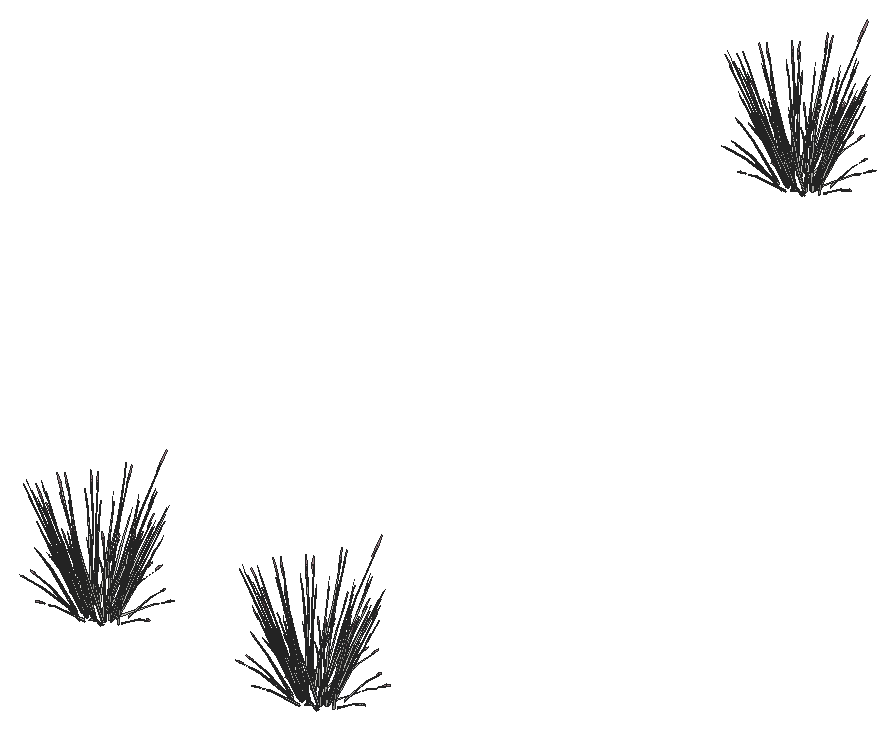
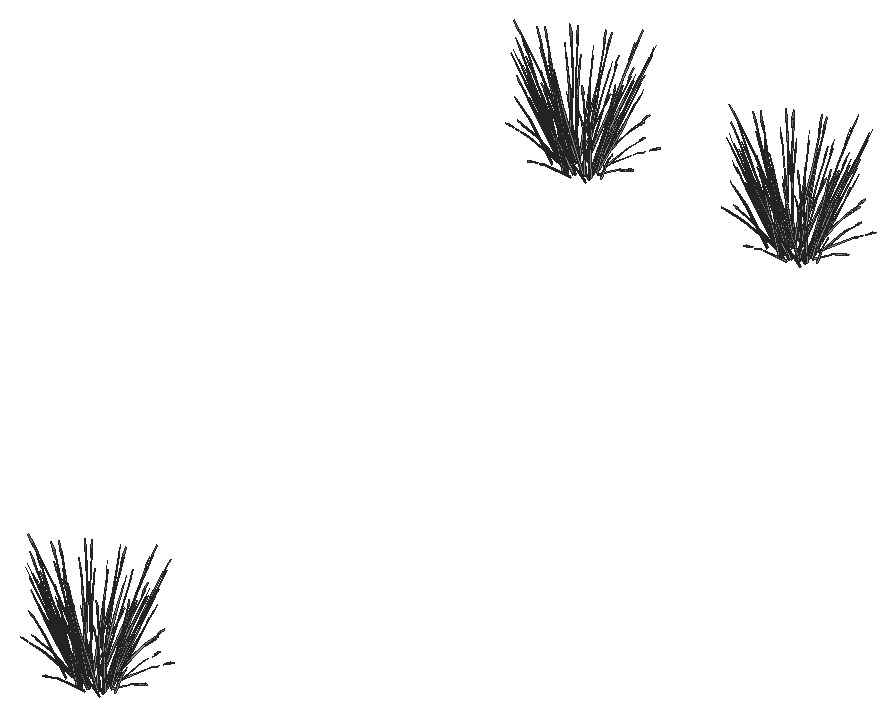
# SketchUp Ruby script. Lengths in millimetres.
U = 1.mm
M = Sketchup.active_model
def pt(a) = Geom::Point3d.new(a.map { |v| v * U })
def face(e, loops, mat)
  f = e.add_face(loops[0].map { |a| pt(a) })
  loops[1..].each { |l| e.add_face(l.map { |a| pt(a) }).erase! }
  f.material = f.back_material = mat if mat
  f
end
# faces: each face lists its corners as indices into pts; further lists are holes
def faces(e, pts, list, mat = nil) = list.each { |f| face(e, (f[0].is_a?(Array) ? f : [f]).map { |l| l.map { |i| pts[i] } }, mat) }
# xy, xz, yz: faces in a plane at the given z, y or x. An outline is a flat list of corners, or four numbers for a rectangle; further outlines are holes
def ring(l) = l.size == 4 ? [[l[0], l[1]], [l[2], l[1]], [l[2], l[3]], [l[0], l[3]]] : l.each_slice(2).to_a
def flat(e, list, mat, &to3) = list.each { |f| face(e, (f[0].is_a?(Array) ? f : [f]).map { |l| ring(l).map { |u, v| to3.(u, v) } }, mat) }
def xy(e, z, list, mat = nil) = flat(e, list, mat) { |x, y| [x, y, z] }
def xz(e, y, list, mat = nil) = flat(e, list, mat) { |x, z| [x, y, z] }
def yz(e, x, list, mat = nil) = flat(e, list, mat) { |y, z| [x, y, z] }
def lines(e, pts, list) = list.each { |a, b| e.add_line(pt(pts[a]), pt(pts[b])) }
# prism: a flat outline (further loops are holes) pulled along v
def prism(e, loops, v, mat = nil)
  f = face(e, loops, mat); d = Geom::Vector3d.new(v.map { |x| x * U })
  f.pushpull(f.normal.samedirection?(d) ? d.length : -d.length)
end
def box(e, o, s, mat = nil) = prism(e, [[o, [o[0] + s[0], o[1], o[2]], [o[0] + s[0], o[1] + s[1], o[2]], [o[0], o[1] + s[1], o[2]]]], [0, 0, s[2]], mat)
def at(x, y, z, deg = 0) = Geom::Transformation.translation(pt([x, y, z])) * Geom::Transformation.rotation(ORIGIN, Z_AXIS, deg.degrees)
def axes(o, x, y, z) = Geom::Transformation.new([*x, 0, *y, 0, *z, 0, *pt(o).to_a, 1])
def part(name) = M.definitions.add(name)
# library, detail: a bought-in or finely detailed component or shape, given as its bounding box
def library(name, o, s) = part(name).tap { |d| box(d.entities, o, s) }
def detail(e, o, s) = box(e.add_group.entities, o, s)
def put(e, d, t, mat = nil) = e.add_instance(d, t).tap { |i| i.material = mat if mat }
def group(e, t, mat = nil) = e.add_group.tap { |g| g.transformation = t; g.material = mat if mat }.entities
root = M.entities
M.materials.add("LightPink_Translucent").color = [144, 107, 117]
M.materials["LightPink_Translucent"].alpha = 0.8
c1 = part("blade")
p = [[54.7,5.3,558.8],[0,4.4,0],[2.3,11.5,0],[55.5,7.8,558.8],[58.2,7.8,558.8],[9.8,11.5,0],
  [62.9,5.7,838.2],[63,6,838.2],[63.4,6,838.2]]
faces(c1.entities,p,[[0,1,2,3],[4,5,2,3],[6,0,3,7],[7,3,4,8]])
c2 = part("seeds")
p = [[7.6,-2.7,35.1],[-0.2,-0.6,40.4],[-0.2,-0.8,0.9],[3.5,-1.8,-1.7],[7.5,-0.8,76.3],[3.7,0.2,78.9]]
faces(c2.entities,p,[[0,1,2,3],[1,0,4,5]],"LightPink_Translucent")
c3 = part("blade with seeds")
put(c3.entities,c1,at(0,0,0))
put(c3.entities,c2,axes([60.9,6.5,787.2],[1.5799,-0.05474,1.17369],[-0.12525,1.92788,0.29478],[-0.07173,-0.02425,1.56792]))
put(root,c3,axes([14274.4,4445.5,8532.4],[0.06562,-1.05324,-0.1216],[1.2424,0.02879,-0.67495],[0.4785,0.07316,1.02557]))
put(root,c3,axes([14038.3,4342.9,8532.4],[0.6166,0.93779,-0.1216],[-1.09436,0.46085,-0.67495],[-0.46117,0.12373,1.02557]))
put(root,c3,axes([14271.2,4290.9,8532.4],[-1.34686,-0.05131,-0.1216],[0.03681,-0.97156,-0.67495],[0.09356,-0.37418,1.02557]))
put(root,c3,axes([14309.6,4396.1,8532.4],[-0.6166,-0.93779,-0.1216],[1.09436,-0.46085,-0.67495],[0.46117,-0.12373,1.02557]))
put(root,c3,axes([14139.9,4475.6,8532.4],[1.19922,-0.48218,-0.1216],[0.58932,0.85579,-0.67495],[0.15822,0.36063,1.02557]))
put(root,c3,axes([14073.5,4293.4,8532.4],[-0.06562,1.05324,-0.1216],[-1.2424,-0.02879,-0.67495],[-0.4785,-0.07316,1.02557]))
put(root,c3,axes([14212.3,4474.6,8532.4],[0.73026,-0.88648,-0.1216],[1.05755,0.51071,-0.67495],[0.36761,0.25045,1.02557]))
put(root,c3,axes([14039.4,4399.5,8532.4],[1.1336,0.57106,-0.1216],[-0.65308,0.827,-0.67495],[-0.32027,0.28747,1.02557]))
put(root,c3,axes([14208,4263.4,8532.4],[-1.19922,0.48218,-0.1216],[-0.58932,-0.85579,-0.67495],[-0.15822,-0.36063,1.02557]))
put(root,c3,axes([14308.5,4339.4,8532.4],[-1.1336,-0.57106,-0.1216],[0.65308,-0.827,-0.67495],[0.32027,-0.28747,1.02557]))
put(root,c3,axes([16302.6,4445.5,8532.4],[0.06562,-1.05324,-0.1216],[1.2424,0.02879,-0.67495],[0.4785,0.07316,1.02557]))
put(root,c3,axes([16066.4,4342.9,8532.4],[0.6166,0.93779,-0.1216],[-1.09436,0.46085,-0.67495],[-0.46117,0.12373,1.02557]))
put(root,c3,axes([16299.4,4290.9,8532.4],[-1.34686,-0.05131,-0.1216],[0.03681,-0.97156,-0.67495],[0.09356,-0.37418,1.02557]))
put(root,c3,axes([16337.8,4396.1,8532.4],[-0.6166,-0.93779,-0.1216],[1.09436,-0.46085,-0.67495],[0.46117,-0.12373,1.02557]))
put(root,c3,axes([16168.1,4475.6,8532.4],[1.19922,-0.48218,-0.1216],[0.58932,0.85579,-0.67495],[0.15822,0.36063,1.02557]))
put(root,c3,axes([16101.6,4293.4,8532.4],[-0.06562,1.05324,-0.1216],[-1.2424,-0.02879,-0.67495],[-0.4785,-0.07316,1.02557]))
put(root,c3,axes([16240.5,4474.6,8532.4],[0.73026,-0.88648,-0.1216],[1.05755,0.51071,-0.67495],[0.36761,0.25045,1.02557]))
put(root,c3,axes([16067.6,4399.5,8532.4],[1.1336,0.57106,-0.1216],[-0.65308,0.827,-0.67495],[-0.32027,0.28747,1.02557]))
put(root,c3,axes([16236.1,4263.4,8532.4],[-1.19922,0.48218,-0.1216],[-0.58932,-0.85579,-0.67495],[-0.15822,-0.36063,1.02557]))
put(root,c3,axes([16336.6,4339.4,8532.4],[-1.1336,-0.57106,-0.1216],[0.65308,-0.827,-0.67495],[0.32027,-0.28747,1.02557]))
put(root,c3,axes([14274.4,12692.7,8532.4],[0.06562,-1.05324,-0.1216],[1.2424,0.02879,-0.67495],[0.4785,0.07316,1.02557]))
put(root,c3,axes([14038.3,12590,8532.4],[0.6166,0.93779,-0.1216],[-1.09436,0.46085,-0.67495],[-0.46117,0.12373,1.02557]))
put(root,c3,axes([14271.2,12538,8532.4],[-1.34686,-0.05131,-0.1216],[0.03681,-0.97156,-0.67495],[0.09356,-0.37418,1.02557]))
put(root,c3,axes([14309.6,12643.2,8532.4],[-0.6166,-0.93779,-0.1216],[1.09436,-0.46085,-0.67495],[0.46117,-0.12373,1.02557]))
put(root,c3,axes([14139.9,12722.7,8532.4],[1.19922,-0.48218,-0.1216],[0.58932,0.85579,-0.67495],[0.15822,0.36063,1.02557]))
put(root,c3,axes([14073.5,12540.5,8532.4],[-0.06562,1.05324,-0.1216],[-1.2424,-0.02879,-0.67495],[-0.4785,-0.07316,1.02557]))
put(root,c3,axes([14212.3,12721.8,8532.4],[0.73026,-0.88648,-0.1216],[1.05755,0.51071,-0.67495],[0.36761,0.25045,1.02557]))
put(root,c3,axes([14039.4,12646.6,8532.4],[1.1336,0.57106,-0.1216],[-0.65308,0.827,-0.67495],[-0.32027,0.28747,1.02557]))
put(root,c3,axes([14208,12510.5,8532.4],[-1.19922,0.48218,-0.1216],[-0.58932,-0.85579,-0.67495],[-0.15822,-0.36063,1.02557]))
put(root,c3,axes([14308.5,12586.6,8532.4],[-1.1336,-0.57106,-0.1216],[0.65308,-0.827,-0.67495],[0.32027,-0.28747,1.02557]))
put(root,c3,axes([14233.3,4341.8,8518.1],[-1.05895,-0.53811,1.38283],[1.11816,-0.83781,0.59665],[0.34166,0.5049,1.33663]))
put(root,c3,axes([16261.5,4341.8,8518.1],[-1.05895,-0.53811,1.38283],[1.11816,-0.83781,0.59665],[0.34166,0.5049,1.33663]))
put(root,c3,axes([14233.3,12588.9,8518.1],[-1.05895,-0.53811,1.38283],[1.11816,-0.83781,0.59665],[0.34166,0.5049,1.33663]))
put(root,c3,axes([14005.6,4366.6,8524.3],[-0.20012,0.13446,1.74944],[0.01702,0.98243,-0.27667],[-0.45871,0.12776,0.14031]))
put(root,c3,axes([14394.7,4358.7,8524.3],[0.17006,-0.15775,1.74944],[-0.21766,-0.96766,-0.27667],[0.42669,-0.18347,0.14031]))
put(root,c3,axes([14301.9,4429.5,8524.3],[0.26289,-0.01751,1.74944],[0.72108,-0.8046,-0.27667],[0.46761,0.10621,0.14031]))
put(root,c3,axes([14302.3,4251.7,8524.3],[-0.01183,-0.20612,1.74944],[-0.99913,-0.59572,-0.27667],[0.15447,-0.36112,0.14031]))
put(root,c3,axes([14006.4,4459.8,8524.3],[-0.03046,0.20495,1.74944],[0.86449,0.71297,-0.27667],[-0.22632,0.33716,0.14031]))
put(root,c3,axes([14132.8,4524.2,8524.3],[0.15534,0.16677,1.74944],[1.25362,0.06552,-0.27667],[0.12606,0.3678,0.14031]))
put(root,c3,axes([14159.6,4206.4,8524.3],[-0.18744,-0.14521,1.74944],[-1.25089,0.09206,-0.27667],[-0.19964,-0.34731,0.14031]))
put(root,c3,axes([14055.4,4247,8524.3],[-0.26368,-0.00731,1.74944],[-0.83946,0.73103,-0.27667],[-0.44791,-0.14937,0.14031]))
put(root,c3,axes([16033.7,4366.6,8524.3],[-0.20012,0.13446,1.74944],[0.01702,0.98243,-0.27667],[-0.45871,0.12776,0.14031]))
put(root,c3,axes([16422.8,4358.7,8524.3],[0.17006,-0.15775,1.74944],[-0.21766,-0.96766,-0.27667],[0.42669,-0.18347,0.14031]))
put(root,c3,axes([16330,4429.5,8524.3],[0.26289,-0.01751,1.74944],[0.72108,-0.8046,-0.27667],[0.46761,0.10621,0.14031]))
put(root,c3,axes([16330.5,4251.7,8524.3],[-0.01183,-0.20612,1.74944],[-0.99913,-0.59572,-0.27667],[0.15447,-0.36112,0.14031]))
put(root,c3,axes([16034.6,4459.8,8524.3],[-0.03046,0.20495,1.74944],[0.86449,0.71297,-0.27667],[-0.22632,0.33716,0.14031]))
put(root,c3,axes([16160.9,4524.2,8524.3],[0.15534,0.16677,1.74944],[1.25362,0.06552,-0.27667],[0.12606,0.3678,0.14031]))
put(root,c3,axes([16187.8,4206.4,8524.3],[-0.18744,-0.14521,1.74944],[-1.25089,0.09206,-0.27667],[-0.19964,-0.34731,0.14031]))
put(root,c3,axes([16083.6,4247,8524.3],[-0.26368,-0.00731,1.74944],[-0.83946,0.73103,-0.27667],[-0.44791,-0.14937,0.14031]))
put(root,c3,axes([14005.6,12613.8,8524.3],[-0.20012,0.13446,1.74944],[0.01702,0.98243,-0.27667],[-0.45871,0.12776,0.14031]))
put(root,c3,axes([14394.7,12605.8,8524.3],[0.17006,-0.15775,1.74944],[-0.21766,-0.96766,-0.27667],[0.42669,-0.18347,0.14031]))
put(root,c3,axes([14301.9,12676.6,8524.3],[0.26289,-0.01751,1.74944],[0.72108,-0.8046,-0.27667],[0.46761,0.10621,0.14031]))
put(root,c3,axes([14302.3,12498.8,8524.3],[-0.01183,-0.20612,1.74944],[-0.99913,-0.59572,-0.27667],[0.15447,-0.36112,0.14031]))
put(root,c3,axes([14006.4,12706.9,8524.3],[-0.03046,0.20495,1.74944],[0.86449,0.71297,-0.27667],[-0.22632,0.33716,0.14031]))
put(root,c3,axes([14132.8,12771.3,8524.3],[0.15534,0.16677,1.74944],[1.25362,0.06552,-0.27667],[0.12606,0.3678,0.14031]))
put(root,c3,axes([14159.6,12453.6,8524.3],[-0.18744,-0.14521,1.74944],[-1.25089,0.09206,-0.27667],[-0.19964,-0.34731,0.14031]))
put(root,c3,axes([14055.4,12494.2,8524.3],[-0.26368,-0.00731,1.74944],[-0.83946,0.73103,-0.27667],[-0.44791,-0.14937,0.14031]))
put(root,c3,axes([14029.7,4262.8,8524.1],[0.09085,0.10335,1.77383],[-0.43798,0.92907,-0.16761],[-0.44357,0.00672,0.31391]))
put(root,c3,axes([14127,4194.3,8524.1],[-0.02286,0.12414,1.77383],[-1.12758,0.45052,-0.16761],[-0.33182,-0.23029,0.31391]))
put(root,c3,axes([14188.1,4493.3,8524.1],[0.00363,-0.12539,1.77383],[1.0502,-0.55319,-0.16761],[0.36479,0.19745,0.31391]))
put(root,c3,axes([13949.1,4391.9,8524.1],[0.1564,0.02778,1.77383],[0.48382,0.91506,-0.16761],[-0.32016,0.24017,0.31391]))
put(root,c3,axes([14379.4,4333.2,8524.1],[-0.16006,-0.00787,1.77383],[-0.66468,-0.8428,-0.16761],[0.26693,-0.27711,0.31391]))
put(root,c3,axes([14371.9,4466.8,8524.1],[-0.11081,-0.09067,1.77383],[0.2424,-0.97188,-0.16761],[0.43649,-0.06209,0.31391]))
put(root,c3,axes([14004,4513.2,8524.1],[0.13903,-0.06253,1.77383],[1.14912,0.41591,-0.16761],[-0.027,0.34629,0.31391]))
put(root,c3,axes([14295.6,4232.8,8524.1],[-0.12446,0.07911,1.77383],[-1.21937,-0.26689,-0.16761],[-0.04414,-0.34521,0.31391]))
put(root,c3,axes([16057.8,4262.8,8524.1],[0.09085,0.10335,1.77383],[-0.43798,0.92907,-0.16761],[-0.44357,0.00672,0.31391]))
put(root,c3,axes([16155.2,4194.3,8524.1],[-0.02286,0.12414,1.77383],[-1.12758,0.45052,-0.16761],[-0.33182,-0.23029,0.31391]))
put(root,c3,axes([16216.2,4493.3,8524.1],[0.00363,-0.12539,1.77383],[1.0502,-0.55319,-0.16761],[0.36479,0.19745,0.31391]))
put(root,c3,axes([15977.3,4391.9,8524.1],[0.1564,0.02778,1.77383],[0.48382,0.91506,-0.16761],[-0.32016,0.24017,0.31391]))
put(root,c3,axes([16407.5,4333.2,8524.1],[-0.16006,-0.00787,1.77383],[-0.66468,-0.8428,-0.16761],[0.26693,-0.27711,0.31391]))
put(root,c3,axes([16400.1,4466.8,8524.1],[-0.11081,-0.09067,1.77383],[0.2424,-0.97188,-0.16761],[0.43649,-0.06209,0.31391]))
put(root,c3,axes([16032.1,4513.2,8524.1],[0.13903,-0.06253,1.77383],[1.14912,0.41591,-0.16761],[-0.027,0.34629,0.31391]))
put(root,c3,axes([16323.7,4232.8,8524.1],[-0.12446,0.07911,1.77383],[-1.21937,-0.26689,-0.16761],[-0.04414,-0.34521,0.31391]))
put(root,c3,axes([14029.7,12509.9,8524.1],[0.09085,0.10335,1.77383],[-0.43798,0.92907,-0.16761],[-0.44357,0.00672,0.31391]))
put(root,c3,axes([14127,12441.5,8524.1],[-0.02286,0.12414,1.77383],[-1.12758,0.45052,-0.16761],[-0.33182,-0.23029,0.31391]))
put(root,c3,axes([14188.1,12740.5,8524.1],[0.00363,-0.12539,1.77383],[1.0502,-0.55319,-0.16761],[0.36479,0.19745,0.31391]))
put(root,c3,axes([13949.1,12639,8524.1],[0.1564,0.02778,1.77383],[0.48382,0.91506,-0.16761],[-0.32016,0.24017,0.31391]))
put(root,c3,axes([14379.4,12580.3,8524.1],[-0.16006,-0.00787,1.77383],[-0.66468,-0.8428,-0.16761],[0.26693,-0.27711,0.31391]))
put(root,c3,axes([14371.9,12713.9,8524.1],[-0.11081,-0.09067,1.77383],[0.2424,-0.97188,-0.16761],[0.43649,-0.06209,0.31391]))
put(root,c3,axes([14004,12760.3,8524.1],[0.13903,-0.06253,1.77383],[1.14912,0.41591,-0.16761],[-0.027,0.34629,0.31391]))
put(root,c3,axes([14295.6,12480,8524.1],[-0.12446,0.07911,1.77383],[-1.21937,-0.26689,-0.16761],[-0.04414,-0.34521,0.31391]))
put(root,c3,axes([14076.7,4448,8541.6],[1.34686,0.05131,-0.13498],[-0.03681,0.97156,-0.74919],[-0.09356,0.37418,1.13838]))
put(root,c3,axes([16104.8,4448,8541.6],[1.34686,0.05131,-0.13498],[-0.03681,0.97156,-0.74919],[-0.09356,0.37418,1.13838]))
put(root,c3,axes([14076.7,12695.2,8541.6],[1.34686,0.05131,-0.13498],[-0.03681,0.97156,-0.74919],[-0.09356,0.37418,1.13838]))
put(root,c3,axes([14135.1,4254.3,8542.4],[-0.81789,0.99285,-0.13619],[-1.18445,-0.572,-0.75594],[-0.41173,-0.28051,1.14864]))
put(root,c3,axes([16163.2,4254.3,8542.4],[-0.81789,0.99285,-0.13619],[-1.18445,-0.572,-0.75594],[-0.41173,-0.28051,1.14864]))
put(root,c3,axes([14135.1,12501.4,8542.4],[-0.81789,0.99285,-0.13619],[-1.18445,-0.572,-0.75594],[-0.41173,-0.28051,1.14864]))
put(root,c3,axes([14128.7,4256,8524.7],[0.55698,-0.6579,0.0643],[0.79316,0.38303,0.50621],[-0.25643,-0.21093,0.77189]))
put(root,c3,axes([14140.6,4485.4,8524.7],[-0.90301,0.35198,0.0643],[-0.44199,-0.64184,0.50621],[0.08721,0.28293,0.77189]))
put(root,c3,axes([14319,4334.1,8524.7],[0.8413,0.43556,0.0643],[-0.48981,0.62025,0.50621],[0.26973,-0.20053,0.77189]))
put(root,c3,axes([14322.2,4395.5,8524.7],[0.4501,0.70615,0.0643],[-0.82077,0.34564,0.50621],[0.36181,-0.0682,0.77189]))
put(root,c3,axes([14062.3,4288.9,8524.7],[0.06171,-0.78753,0.0643],[0.9318,0.02159,0.50621],[-0.35694,-0.08241,0.77189]))
put(root,c3,axes([14276.9,4282.1,8524.7],[1.00708,0.04826,0.0643],[-0.02761,0.72867,0.50621],[0.10538,-0.27912,0.77189]))
put(root,c3,axes([14285.7,4450,8524.7],[-0.06171,0.78753,0.0643],[-0.9318,-0.02159,0.50621],[0.35694,0.08241,0.77189]))
put(root,c3,axes([14028.9,4404.8,8524.7],[-0.8413,-0.43556,0.0643],[0.48981,-0.62025,0.50621],[-0.26973,0.20053,0.77189]))
put(root,c3,axes([14207.3,4253.5,8524.7],[0.90301,-0.35198,0.0643],[0.44199,0.64184,0.50621],[-0.08721,-0.28293,0.77189]))
put(root,c3,axes([14025.7,4343.4,8524.7],[-0.4501,-0.70615,0.0643],[0.82077,-0.34564,0.50621],[-0.36181,0.0682,0.77189]))
put(root,c3,axes([14219.2,4482.9,8524.7],[-0.55698,0.6579,0.0643],[-0.79316,-0.38303,0.50621],[0.25643,0.21093,0.77189]))
put(root,c3,axes([14071,4456.8,8524.7],[-1.00708,-0.04826,0.0643],[0.02761,-0.72867,0.50621],[-0.10538,0.27912,0.77189]))
put(root,c3,axes([16156.9,4256,8524.7],[0.55698,-0.6579,0.0643],[0.79316,0.38303,0.50621],[-0.25643,-0.21093,0.77189]))
put(root,c3,axes([16168.8,4485.4,8524.7],[-0.90301,0.35198,0.0643],[-0.44199,-0.64184,0.50621],[0.08721,0.28293,0.77189]))
put(root,c3,axes([16347.1,4334.1,8524.7],[0.8413,0.43556,0.0643],[-0.48981,0.62025,0.50621],[0.26973,-0.20053,0.77189]))
put(root,c3,axes([16350.3,4395.5,8524.7],[0.4501,0.70615,0.0643],[-0.82077,0.34564,0.50621],[0.36181,-0.0682,0.77189]))
put(root,c3,axes([16090.4,4288.9,8524.7],[0.06171,-0.78753,0.0643],[0.9318,0.02159,0.50621],[-0.35694,-0.08241,0.77189]))
put(root,c3,axes([16305.1,4282.1,8524.7],[1.00708,0.04826,0.0643],[-0.02761,0.72867,0.50621],[0.10538,-0.27912,0.77189]))
put(root,c3,axes([16313.8,4450,8524.7],[-0.06171,0.78753,0.0643],[-0.9318,-0.02159,0.50621],[0.35694,0.08241,0.77189]))
put(root,c3,axes([16057.1,4404.8,8524.7],[-0.8413,-0.43556,0.0643],[0.48981,-0.62025,0.50621],[-0.26973,0.20053,0.77189]))
put(root,c3,axes([16235.4,4253.5,8524.7],[0.90301,-0.35198,0.0643],[0.44199,0.64184,0.50621],[-0.08721,-0.28293,0.77189]))
put(root,c3,axes([16053.9,4343.4,8524.7],[-0.4501,-0.70615,0.0643],[0.82077,-0.34564,0.50621],[-0.36181,0.0682,0.77189]))
put(root,c3,axes([16247.3,4482.9,8524.7],[-0.55698,0.6579,0.0643],[-0.79316,-0.38303,0.50621],[0.25643,0.21093,0.77189]))
put(root,c3,axes([16099.1,4456.8,8524.7],[-1.00708,-0.04826,0.0643],[0.02761,-0.72867,0.50621],[-0.10538,0.27912,0.77189]))
put(root,c3,axes([14128.7,12503.2,8524.7],[0.55698,-0.6579,0.0643],[0.79316,0.38303,0.50621],[-0.25643,-0.21093,0.77189]))
put(root,c3,axes([14140.6,12732.5,8524.7],[-0.90301,0.35198,0.0643],[-0.44199,-0.64184,0.50621],[0.08721,0.28293,0.77189]))
put(root,c3,axes([14319,12581.2,8524.7],[0.8413,0.43556,0.0643],[-0.48981,0.62025,0.50621],[0.26973,-0.20053,0.77189]))
put(root,c3,axes([14322.2,12642.7,8524.7],[0.4501,0.70615,0.0643],[-0.82077,0.34564,0.50621],[0.36181,-0.0682,0.77189]))
put(root,c3,axes([14062.3,12536.1,8524.7],[0.06171,-0.78753,0.0643],[0.9318,0.02159,0.50621],[-0.35694,-0.08241,0.77189]))
put(root,c3,axes([14276.9,12529.2,8524.7],[1.00708,0.04826,0.0643],[-0.02761,0.72867,0.50621],[0.10538,-0.27912,0.77189]))
put(root,c3,axes([14285.7,12697.1,8524.7],[-0.06171,0.78753,0.0643],[-0.9318,-0.02159,0.50621],[0.35694,0.08241,0.77189]))
put(root,c3,axes([14028.9,12652,8524.7],[-0.8413,-0.43556,0.0643],[0.48981,-0.62025,0.50621],[-0.26973,0.20053,0.77189]))
put(root,c3,axes([14207.3,12500.7,8524.7],[0.90301,-0.35198,0.0643],[0.44199,0.64184,0.50621],[-0.08721,-0.28293,0.77189]))
put(root,c3,axes([14025.7,12590.5,8524.7],[-0.4501,-0.70615,0.0643],[0.82077,-0.34564,0.50621],[-0.36181,0.0682,0.77189]))
put(root,c3,axes([14219.2,12730,8524.7],[-0.55698,0.6579,0.0643],[-0.79316,-0.38303,0.50621],[0.25643,0.21093,0.77189]))
put(root,c3,axes([14071,12703.9,8524.7],[-1.00708,-0.04826,0.0643],[0.02761,-0.72867,0.50621],[-0.10538,0.27912,0.77189]))
put(root,c3,axes([14199.1,4255.3,8524.7],[1.20755,0.27075,0.48003],[-0.41292,0.89013,0.3958],[-0.07257,-0.35005,0.9933]))
put(root,c3,axes([14287.8,4443.6,8524.7],[-0.90362,0.68241,0.48003],[-0.77932,-0.72471,0.3958],[0.42395,0.12588,0.9933]))
put(root,c3,axes([14320,4389.2,8524.7],[-0.34623,0.9443,0.48003],[-1.13828,-0.3229,0.3958],[0.44763,-0.05675,0.9933]))
put(root,c3,axes([14034.9,4409.5,8524.7],[-0.30393,-0.95317,0.48003],[1.19224,-0.16542,0.3958],[-0.35138,0.22417,0.9933]))
put(root,c3,axes([14079.1,4458.5,8524.7],[-0.87265,-0.70663,0.48003],[0.92674,-0.60943,0.3958],[-0.16097,0.33153,0.9933]))
put(root,c3,axes([14268.8,4280.4,8524.7],[0.87265,0.70663,0.48003],[-0.92674,0.60943,0.3958],[0.16097,-0.33153,0.9933]))
put(root,c3,axes([14027.9,4349.8,8524.7],[0.34623,-0.9443,0.48003],[1.13828,0.3229,0.3958],[-0.44763,0.05675,0.9933]))
put(root,c3,axes([14313,4329.4,8524.7],[0.30393,0.95317,0.48003],[-1.19224,0.16542,0.3958],[0.35138,-0.22417,0.9933]))
put(root,c3,axes([14225.1,4478.2,8524.7],[-1.21888,0.23767,0.48003],[-0.21154,-0.93233,0.3958],[0.28666,0.27478,0.9933]))
put(root,c3,axes([16227.3,4255.3,8524.7],[1.20755,0.27075,0.48003],[-0.41292,0.89013,0.3958],[-0.07257,-0.35005,0.9933]))
put(root,c3,axes([16316,4443.6,8524.7],[-0.90362,0.68241,0.48003],[-0.77932,-0.72471,0.3958],[0.42395,0.12588,0.9933]))
put(root,c3,axes([16348.1,4389.2,8524.7],[-0.34623,0.9443,0.48003],[-1.13828,-0.3229,0.3958],[0.44763,-0.05675,0.9933]))
put(root,c3,axes([16063,4409.5,8524.7],[-0.30393,-0.95317,0.48003],[1.19224,-0.16542,0.3958],[-0.35138,0.22417,0.9933]))
put(root,c3,axes([16107.3,4458.5,8524.7],[-0.87265,-0.70663,0.48003],[0.92674,-0.60943,0.3958],[-0.16097,0.33153,0.9933]))
put(root,c3,axes([16296.9,4280.4,8524.7],[0.87265,0.70663,0.48003],[-0.92674,0.60943,0.3958],[0.16097,-0.33153,0.9933]))
put(root,c3,axes([16056.1,4349.8,8524.7],[0.34623,-0.9443,0.48003],[1.13828,0.3229,0.3958],[-0.44763,0.05675,0.9933]))
put(root,c3,axes([16341.2,4329.4,8524.7],[0.30393,0.95317,0.48003],[-1.19224,0.16542,0.3958],[0.35138,-0.22417,0.9933]))
put(root,c3,axes([16253.3,4478.2,8524.7],[-1.21888,0.23767,0.48003],[-0.21154,-0.93233,0.3958],[0.28666,0.27478,0.9933]))
put(root,c3,axes([14199.1,12502.4,8524.7],[1.20755,0.27075,0.48003],[-0.41292,0.89013,0.3958],[-0.07257,-0.35005,0.9933]))
put(root,c3,axes([14287.8,12690.7,8524.7],[-0.90362,0.68241,0.48003],[-0.77932,-0.72471,0.3958],[0.42395,0.12588,0.9933]))
put(root,c3,axes([14320,12636.3,8524.7],[-0.34623,0.9443,0.48003],[-1.13828,-0.3229,0.3958],[0.44763,-0.05675,0.9933]))
put(root,c3,axes([14034.9,12656.6,8524.7],[-0.30393,-0.95317,0.48003],[1.19224,-0.16542,0.3958],[-0.35138,0.22417,0.9933]))
put(root,c3,axes([14079.1,12705.6,8524.7],[-0.87265,-0.70663,0.48003],[0.92674,-0.60943,0.3958],[-0.16097,0.33153,0.9933]))
put(root,c3,axes([14268.8,12527.5,8524.7],[0.87265,0.70663,0.48003],[-0.92674,0.60943,0.3958],[0.16097,-0.33153,0.9933]))
put(root,c3,axes([14027.9,12596.9,8524.7],[0.34623,-0.9443,0.48003],[1.13828,0.3229,0.3958],[-0.44763,0.05675,0.9933]))
put(root,c3,axes([14313,12576.6,8524.7],[0.30393,0.95317,0.48003],[-1.19224,0.16542,0.3958],[0.35138,-0.22417,0.9933]))
put(root,c3,axes([14225.1,12725.3,8524.7],[-1.21888,0.23767,0.48003],[-0.21154,-0.93233,0.3958],[0.28666,0.27478,0.9933]))
put(root,c3,axes([14149.1,4467,8532.8],[0.36946,-0.79643,0.35414],[1.07787,0.23229,-0.4572],[0.09883,0.32066,0.87481]))
put(root,c3,axes([14198.8,4271.9,8532.8],[-0.36946,0.79643,0.35414],[-1.07787,-0.23229,-0.4572],[-0.09883,-0.32066,0.87481]))
put(root,c3,axes([14269.6,4435.1,8532.8],[-0.69728,-0.64842,0.35414],[0.79619,-0.61382,-0.4572],[0.40453,0.09339,0.87481]))
put(root,c3,axes([14298.7,4388.9,8532.8],[-1.01846,-0.28891,0.35414],[0.29705,-0.84289,-0.4572],[0.41005,-0.07729,0.87481]))
put(root,c3,axes([14078.3,4303.9,8532.8],[0.69728,0.64842,0.35414],[-0.79619,0.61382,-0.4572],[-0.40453,-0.09339,0.87481]))
put(root,c3,axes([14090.1,4444.3,8532.8],[0.82919,-0.54528,0.35414],[0.78493,0.62262,-0.4572],[-0.11943,0.31634,0.87481]))
put(root,c3,axes([14053.5,4401.4,8532.8],[1.06674,-0.14801,0.35414],[0.28168,0.84611,-0.4572],[-0.30569,0.22726,0.87481]))
put(root,c3,axes([14214.8,4463.7,8532.8],[-0.18927,-0.83419,0.35414],[1.08199,-0.22027,-0.4572],[0.29062,0.23905,0.87481]))
put(root,c3,axes([14294.4,4337.5,8532.8],[-1.06674,0.14801,0.35414],[-0.28168,-0.84611,-0.4572],[0.30569,-0.22726,0.87481]))
put(root,c3,axes([14049.2,4350,8532.8],[1.01846,0.28891,0.35414],[-0.29705,0.84289,-0.4572],[-0.41005,0.07729,0.87481]))
put(root,c3,axes([14257.8,4294.7,8532.8],[-0.82919,0.54528,0.35414],[-0.78493,-0.62262,-0.4572],[0.11943,-0.31634,0.87481]))
put(root,c3,axes([14133.1,4275.2,8532.8],[0.18927,0.83419,0.35414],[-1.08199,0.22027,-0.4572],[-0.29062,-0.23905,0.87481]))
put(root,c3,axes([16177.3,4467,8532.8],[0.36946,-0.79643,0.35414],[1.07787,0.23229,-0.4572],[0.09883,0.32066,0.87481]))
put(root,c3,axes([16226.9,4271.9,8532.8],[-0.36946,0.79643,0.35414],[-1.07787,-0.23229,-0.4572],[-0.09883,-0.32066,0.87481]))
put(root,c3,axes([16297.8,4435.1,8532.8],[-0.69728,-0.64842,0.35414],[0.79619,-0.61382,-0.4572],[0.40453,0.09339,0.87481]))
put(root,c3,axes([16326.9,4388.9,8532.8],[-1.01846,-0.28891,0.35414],[0.29705,-0.84289,-0.4572],[0.41005,-0.07729,0.87481]))
put(root,c3,axes([16106.5,4303.9,8532.8],[0.69728,0.64842,0.35414],[-0.79619,0.61382,-0.4572],[-0.40453,-0.09339,0.87481]))
put(root,c3,axes([16118.2,4444.3,8532.8],[0.82919,-0.54528,0.35414],[0.78493,0.62262,-0.4572],[-0.11943,0.31634,0.87481]))
put(root,c3,axes([16081.6,4401.4,8532.8],[1.06674,-0.14801,0.35414],[0.28168,0.84611,-0.4572],[-0.30569,0.22726,0.87481]))
put(root,c3,axes([16243,4463.7,8532.8],[-0.18927,-0.83419,0.35414],[1.08199,-0.22027,-0.4572],[0.29062,0.23905,0.87481]))
put(root,c3,axes([16322.6,4337.5,8532.8],[-1.06674,0.14801,0.35414],[-0.28168,-0.84611,-0.4572],[0.30569,-0.22726,0.87481]))
put(root,c3,axes([16077.3,4350,8532.8],[1.01846,0.28891,0.35414],[-0.29705,0.84289,-0.4572],[-0.41005,0.07729,0.87481]))
put(root,c3,axes([16286,4294.7,8532.8],[-0.82919,0.54528,0.35414],[-0.78493,-0.62262,-0.4572],[0.11943,-0.31634,0.87481]))
put(root,c3,axes([16161.2,4275.2,8532.8],[0.18927,0.83419,0.35414],[-1.08199,0.22027,-0.4572],[-0.29062,-0.23905,0.87481]))
put(root,c3,axes([14149.1,12714.2,8532.8],[0.36946,-0.79643,0.35414],[1.07787,0.23229,-0.4572],[0.09883,0.32066,0.87481]))
put(root,c3,axes([14198.8,12519,8532.8],[-0.36946,0.79643,0.35414],[-1.07787,-0.23229,-0.4572],[-0.09883,-0.32066,0.87481]))
put(root,c3,axes([14269.6,12682.2,8532.8],[-0.69728,-0.64842,0.35414],[0.79619,-0.61382,-0.4572],[0.40453,0.09339,0.87481]))
put(root,c3,axes([14298.7,12636,8532.8],[-1.01846,-0.28891,0.35414],[0.29705,-0.84289,-0.4572],[0.41005,-0.07729,0.87481]))
put(root,c3,axes([14078.3,12551,8532.8],[0.69728,0.64842,0.35414],[-0.79619,0.61382,-0.4572],[-0.40453,-0.09339,0.87481]))
put(root,c3,axes([14090.1,12691.4,8532.8],[0.82919,-0.54528,0.35414],[0.78493,0.62262,-0.4572],[-0.11943,0.31634,0.87481]))
put(root,c3,axes([14053.5,12648.6,8532.8],[1.06674,-0.14801,0.35414],[0.28168,0.84611,-0.4572],[-0.30569,0.22726,0.87481]))
put(root,c3,axes([14214.8,12710.8,8532.8],[-0.18927,-0.83419,0.35414],[1.08199,-0.22027,-0.4572],[0.29062,0.23905,0.87481]))
put(root,c3,axes([14294.4,12584.6,8532.8],[-1.06674,0.14801,0.35414],[-0.28168,-0.84611,-0.4572],[0.30569,-0.22726,0.87481]))
put(root,c3,axes([14049.2,12597.2,8532.8],[1.01846,0.28891,0.35414],[-0.29705,0.84289,-0.4572],[-0.41005,0.07729,0.87481]))
put(root,c3,axes([14257.8,12541.8,8532.8],[-0.82919,0.54528,0.35414],[-0.78493,-0.62262,-0.4572],[0.11943,-0.31634,0.87481]))
put(root,c3,axes([14133.1,12522.4,8532.8],[0.18927,0.83419,0.35414],[-1.08199,0.22027,-0.4572],[-0.29062,-0.23905,0.87481]))
put(root,c3,axes([14148.8,4483.6,8533.1],[-1.20755,-0.27075,0.53283],[0.41292,-0.89013,0.43934],[0.07257,0.35005,1.10256]))
put(root,c3,axes([16176.9,4483.6,8533.1],[-1.20755,-0.27075,0.53283],[0.41292,-0.89013,0.43934],[0.07257,0.35005,1.10256]))
put(root,c3,axes([14148.8,12730.8,8533.1],[-1.20755,-0.27075,0.53283],[0.41292,-0.89013,0.43934],[0.07257,0.35005,1.10256]))
put(root,c3,axes([14050.5,4289,8533.9],[1.01205,-0.7643,0.53763],[0.87284,0.81167,0.4433],[-0.47482,-0.14098,1.11249]))
put(root,c3,axes([14120.7,4250.3,8533.9],[1.36515,-0.26619,0.53763],[0.23692,1.04421,0.4433],[-0.32106,-0.30775,1.11249]))
put(root,c3,axes([16078.7,4289,8533.9],[1.01205,-0.7643,0.53763],[0.87284,0.81167,0.4433],[-0.47482,-0.14098,1.11249]))
put(root,c3,axes([16148.9,4250.3,8533.9],[1.36515,-0.26619,0.53763],[0.23692,1.04421,0.4433],[-0.32106,-0.30775,1.11249]))
put(root,c3,axes([14050.5,12536.2,8533.9],[1.01205,-0.7643,0.53763],[0.87284,0.81167,0.4433],[-0.47482,-0.14098,1.11249]))
put(root,c3,axes([14120.7,12497.4,8533.9],[1.36515,-0.26619,0.53763],[0.23692,1.04421,0.4433],[-0.32106,-0.30775,1.11249]))
put(root,c3,axes([14186,4539.2,8547.9],[0.84686,-0.59414,-0.06488],[0.77596,0.65071,-0.29416],[0.05463,0.18438,0.97024]))
put(root,c3,axes([13992,4462.5,8547.9],[1.08141,0.27645,-0.06488],[-0.33265,0.85086,-0.29416],[-0.17688,0.12919,0.97024]))
put(root,c3,axes([16214.1,4539.2,8547.9],[0.84686,-0.59414,-0.06488],[0.77596,0.65071,-0.29416],[0.05463,0.18438,0.97024]))
put(root,c3,axes([16020.1,4462.5,8547.9],[1.08141,0.27645,-0.06488],[-0.33265,0.85086,-0.29416],[-0.17688,0.12919,0.97024]))
put(root,c3,axes([14186,12786.3,8547.9],[0.84686,-0.59414,-0.06488],[0.77596,0.65071,-0.29416],[0.05463,0.18438,0.97024]))
put(root,c3,axes([13992,12709.6,8547.9],[1.08141,0.27645,-0.06488],[-0.33265,0.85086,-0.29416],[-0.17688,0.12919,0.97024]))
